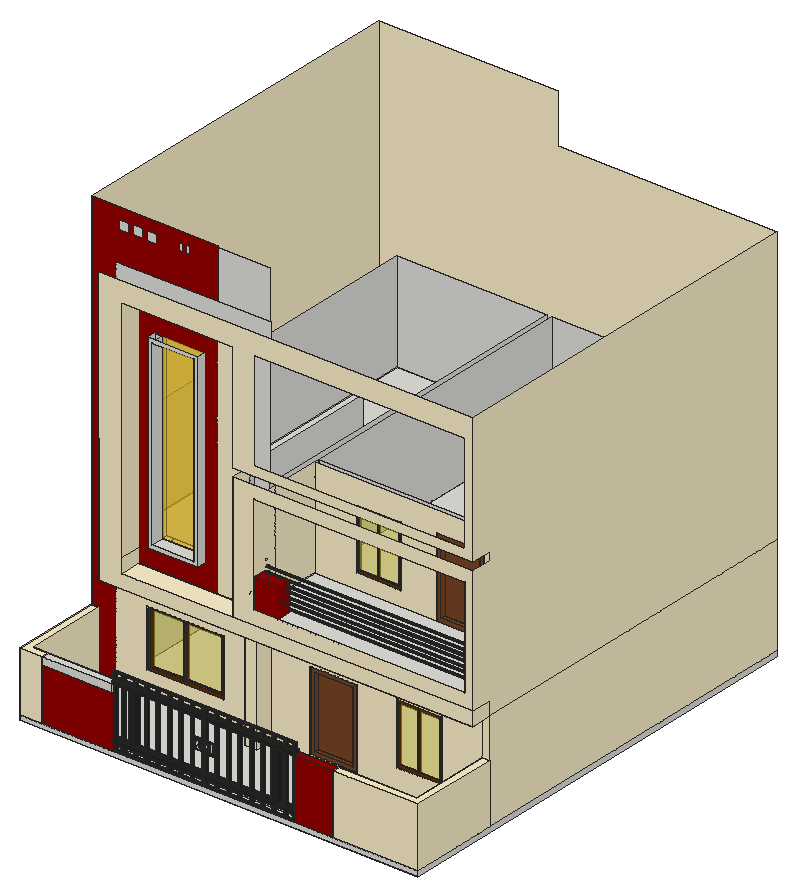
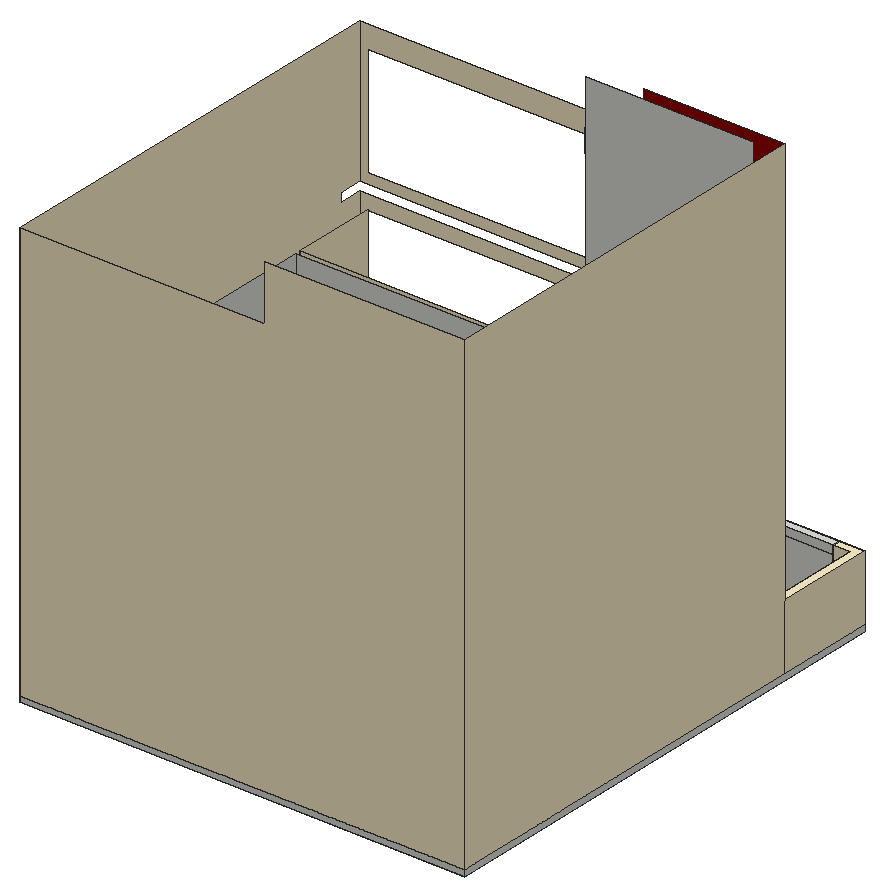
# SketchUp Ruby script. Lengths in inches.
U = 1.inch
M = Sketchup.active_model
def pt(a) = Geom::Point3d.new(a.map { |v| v * U })
def face(e, loops, mat)
  f = e.add_face(loops[0].map { |a| pt(a) })
  loops[1..].each { |l| e.add_face(l.map { |a| pt(a) }).erase! }
  f.material = f.back_material = mat if mat
  f
end
# faces: each face lists its corners as indices into pts; further lists are holes
def faces(e, pts, list, mat = nil) = list.each { |f| face(e, (f[0].is_a?(Array) ? f : [f]).map { |l| l.map { |i| pts[i] } }, mat) }
# xy, xz, yz: faces in a plane at the given z, y or x. An outline is a flat list of corners, or four numbers for a rectangle; further outlines are holes
def ring(l) = l.size == 4 ? [[l[0], l[1]], [l[2], l[1]], [l[2], l[3]], [l[0], l[3]]] : l.each_slice(2).to_a
def flat(e, list, mat, &to3) = list.each { |f| face(e, (f[0].is_a?(Array) ? f : [f]).map { |l| ring(l).map { |u, v| to3.(u, v) } }, mat) }
def xy(e, z, list, mat = nil) = flat(e, list, mat) { |x, y| [x, y, z] }
def xz(e, y, list, mat = nil) = flat(e, list, mat) { |x, z| [x, y, z] }
def yz(e, x, list, mat = nil) = flat(e, list, mat) { |y, z| [x, y, z] }
def lines(e, pts, list) = list.each { |a, b| e.add_line(pt(pts[a]), pt(pts[b])) }
# prism: a flat outline (further loops are holes) pulled along v
def prism(e, loops, v, mat = nil)
  f = face(e, loops, mat); d = Geom::Vector3d.new(v.map { |x| x * U })
  f.pushpull(f.normal.samedirection?(d) ? d.length : -d.length)
end
def box(e, o, s, mat = nil) = prism(e, [[o, [o[0] + s[0], o[1], o[2]], [o[0] + s[0], o[1] + s[1], o[2]], [o[0], o[1] + s[1], o[2]]]], [0, 0, s[2]], mat)
def at(x, y, z, deg = 0) = Geom::Transformation.translation(pt([x, y, z])) * Geom::Transformation.rotation(ORIGIN, Z_AXIS, deg.degrees)
def axes(o, x, y, z) = Geom::Transformation.new([*x, 0, *y, 0, *z, 0, *pt(o).to_a, 1])
def part(name) = M.definitions.add(name)
# library, detail: a bought-in or finely detailed component or shape, given as its bounding box
def library(name, o, s) = part(name).tap { |d| box(d.entities, o, s) }
def detail(e, o, s) = box(e.add_group.entities, o, s)
def put(e, d, t, mat = nil) = e.add_instance(d, t).tap { |i| i.material = mat if mat }
def group(e, t, mat = nil) = e.add_group.tap { |g| g.transformation = t; g.material = mat if mat }.entities
root = M.entities
M.materials.add("[Color A07]").color = [153, 0, 0]
M.materials.add("[Color C08]").color = [102, 51, 0]
M.materials.add("[Color D01]").color = [255, 242, 204]
M.materials.add("[Color M00]").color = [255, 255, 255]
M.materials.add("[Color M09]").color = [0, 0, 0]
M.materials.add("[Metal Corrugated Shiny]").color = [38, 38, 38]
M.materials.add("[Metal Silver]").color = [234, 233, 238]
M.materials.add("[Translucent Glass Blue]").color = [253, 204, 30]
M.materials["[Translucent Glass Blue]"].alpha = 0.5
M.materials.add("[Translucent Glass Gray]").color = [238, 223, 60]
M.materials["[Translucent Glass Gray]"].alpha = 0.5
M.materials.add("[Wood Veneer 01]").color = [120, 70, 37]
c1 = part("Component\#24")
prism(c1.entities,[[[0,1.89,1.72],[0,1.6875,1.91],[0,1.44,2.04],[0,1.18,2.11],[0,0.9,2.11],[0,0.63,2.03],[0,0.39,1.89],[0,0.2,1.6875],[0,0.07,1.44],[0,0,1.18],[0,0,0.9],[0,0.08,0.63],[0,0.22,0.39],[0,0.42,0.2],[0,0.67,0.07],[0,0.9375,0],[0,1.21,0],[0,1.48,0.08],[0,1.72,0.22],[0,1.91,0.42],[0,2.04,0.67],[0,2.11,0.9375],[0,2.11,1.21],[0,2.03,1.48]]],[-0.625,0,0])
c2 = part("Gate cross rail")
box(c2.entities,[0,0,0],[3,48,2])
c3 = part("Gate edge rail")
box(c3.entities,[0,0.5625,0],[48,0.625,0.625])
c4 = part("Gate picket")
box(c4.entities,[0,0,0],[63,1.1875,0.625])
c5 = part("Gate rail")
box(c5.entities,[0,0,0],[3,45,2])
c6 = part("Component\#23")
xy(c6.entities,0,[[0,0,11.01,4.67]])
c7 = part("Gate grille")
put(c7.entities,c2,at(54.625,0,0),"[Metal Corrugated Shiny]")
put(c7.entities,c3,axes([0.625,0,1.96],[0,1,0],[0,0,-1],[-1,0,0]),"[Metal Corrugated Shiny]")
put(c7.entities,c4,at(0.625,46.8125,0.78),"[Metal Corrugated Shiny]")
put(c7.entities,c2,at(6.625,0,0),"[Metal Corrugated Shiny]")
put(c7.entities,c4,at(0.625,10.8125,0.78),"[Metal Corrugated Shiny]")
put(c7.entities,c4,at(0.625,4.8125,0.78),"[Metal Corrugated Shiny]")
put(c7.entities,c3,axes([64.25,0,1.96],[0,1,0],[0,0,-1],[-1,0,0]),"[Metal Corrugated Shiny]")
put(c7.entities,c4,at(0.625,34.8125,0.78),"[Metal Corrugated Shiny]")
put(c7.entities,c4,at(0.625,28.8125,0.78),"[Metal Corrugated Shiny]")
put(c7.entities,c4,at(0.625,40.8125,0.78),"[Metal Corrugated Shiny]")
put(c7.entities,c5,at(9.625,12,0,-90),"[Metal Corrugated Shiny]")
put(c7.entities,c4,at(0.625,22.8125,0.78),"[Metal Corrugated Shiny]")
put(c7.entities,c4,at(0.625,0,0.78),"[Metal Corrugated Shiny]")
put(c7.entities,c4,at(0.625,16.8125,0.78),"[Metal Corrugated Shiny]")
put(c7.entities,c6,axes([26.47,42,1.4],[1,0,0],[0,1.14286,0],[0,0,1]),"[Metal Corrugated Shiny]")
c8 = part("Component\#25")
box(c8.entities,[-0.625,0,0],[0.625,0.9375,5.875])
c9 = part("Forecourt gate leaf")
put(c9.entities,c1,at(0.625,39.09,32.62),"[Metal Silver]")
put(c9.entities,c7,axes([2.03,0,0],[0,0,1],[0,0.875,0],[-1,0,0]))
put(c9.entities,c8,at(0.625,38.15,29.71),"[Metal Silver]")
c10 = part("Group\#2")
xy(c10.entities,0,[[0,0,48,5.9375]],"[Wood Veneer 01]")
xy(c10.entities,4.11,[[4.11,0,43.89,5.9375]],"[Wood Veneer 01]")
xy(c10.entities,79.89,[[4.11,0,43.89,5.9375]],"[Wood Veneer 01]")
xy(c10.entities,84,[[0,0,48,5.9375]],"[Wood Veneer 01]")
xz(c10.entities,0,[[[0,0,48,84],[4.11,4.11,43.89,79.89]]],"[Wood Veneer 01]")
xz(c10.entities,5.9375,[[[0,0,48,84],[4.11,4.11,43.89,79.89]],[4.11,4.11,43.89,79.89]],"[Wood Veneer 01]")
yz(c10.entities,0,[[0,0,5.9375,84]],"[Wood Veneer 01]")
yz(c10.entities,4.11,[[0,4.11,5.9375,79.89]],"[Wood Veneer 01]")
yz(c10.entities,43.89,[[0,4.11,5.9375,79.89]],"[Wood Veneer 01]")
yz(c10.entities,48,[[0,0,5.9375,84]],"[Wood Veneer 01]")
c11 = part("Group\#1")
xy(c11.entities,0,[[0,0,119.6875,5.25]],"[Color C08]")
xy(c11.entities,5.1875,[[5.1875,0,56.1875,5.25],[56.1875,0,59.84,5.25],[59.84,0,114.5,5.25]],"[Color C08]")
xy(c11.entities,114.5,[[5.1875,0,56.1875,5.25],[56.1875,0,59.84,5.25],[59.84,0,114.5,5.25]],"[Color C08]")
xy(c11.entities,119.6875,[[0,0,119.6875,5.25]],"[Color C08]")
xz(c11.entities,0,[[[0,0,119.6875,119.6875],[5.1875,5.1875,114.5,114.5]],[56.1875,5.1875,59.84,114.5]],"[Color C08]")
xz(c11.entities,0,[[5.1875,5.1875,56.1875,114.5],[59.84,5.1875,114.5,114.5]],"[Translucent Glass Gray]")
xz(c11.entities,5.25,[[[0,0,119.6875,119.6875],[5.1875,5.1875,114.5,114.5]],[56.1875,5.1875,59.84,114.5]],"[Color C08]")
yz(c11.entities,0,[[0,0,5.25,119.6875]],"[Color C08]")
yz(c11.entities,5.1875,[[0,5.1875,5.25,114.5]],"[Color C08]")
yz(c11.entities,56.1875,[[0,5.1875,5.25,114.5]],"[Color C08]")
yz(c11.entities,59.84,[[0,5.1875,5.25,114.5]],"[Color C08]")
yz(c11.entities,114.5,[[0,5.1875,5.25,114.5]],"[Color C08]")
yz(c11.entities,119.6875,[[0,0,5.25,119.6875]],"[Color C08]")
xy(root,0,[[0,0.625,480,540.625]])
xy(root,6,[[0,0.625,0,108.25,9,108.25,9,9.625,26.71,9.625,26.71,0.625],[26.71,0.625,110.46,9.625],[110.46,0.625,329.85,9.625],[329.85,0.625,377.41,9.625],[377.41,0.625,377.41,9.625,471,9.625,471,108.25,480,108.25,480,0.625],
  [9,9.625,471,9.625,471,108.25,215.91,108.25,215.91,86.8125,201.94,86.8125,201.94,108.25,9,108.25],[[0,108.25,480,540.625],[216.3125,114.25,471,531.625],[29.875,114.25,210.3125,531.625]],[29.875,114.25,210.3125,531.625],[216.3125,114.25,471,531.625]])
xy(root,8.27,[[262.79,108.25,319.98,114.25]])
xy(root,30.65,[[66.9,108.25,160.09,114.25]])
xy(root,31.26,[[368.53,108.25,422.35,114.25]])
xy(root,68.9375,[[26.71,0.625,110.46,9.625]])
xy(root,78,[[26.71,0.625,110.46,9.625]])
xy(root,78,[[329.85,0.625,377.41,9.625]],"[Color A07]")
xy(root,78,[[0,0.625,26.71,0.625,26.71,9.625,9,9.625,9,108.25,0,108.25],[377.41,0.625,480,0.625,480,108.25,471,108.25,471,9.625,377.41,9.625]],"[Color D01]")
xy(root,100.15,[[66.9,108.25,160.09,114.25]])
xy(root,103.83,[[262.79,108.25,319.98,114.25]])
xy(root,105.07,[[368.53,108.25,422.35,114.25]])
xy(root,126,[[471,82.5625,480,108.25],[201.94,86.8125,215.91,108.25]])
xy(root,126,[[29.875,82.5625,471,82.5625,471,108.25,215.91,108.25,215.91,86.8125,201.94,86.8125,201.94,108.25,29.875,108.25]],"[Color M00]")
xy(root,142.4375,[[191.1875,82.5625,471,108.25],[471,82.5625,480,108.25],[191.1875,108.25,471,278.125]])
xy(root,142.4375,[[56.54,82.5625,191.1875,108.25]],"[Color D01]")
xy(root,152.875,[[29.875,114.25,210.3125,531.625],[216.3125,114.25,471,531.625]])
xy(root,158.875,[[245.1875,82.5625,471,82.5625,471,114.25,216.3125,114.25,216.3125,98.41,245.1875,98.41],[29.875,114.25,210.3125,531.625],[216.3125,114.25,471,114.25,471,173.875,420.42,173.875,420.42,179.875,363.24,179.875,363.24,173.875,216.3125,173.875],[216.3125,173.875,363.24,179.875],[420.42,173.875,471,179.875],
  [216.3125,179.875,471,531.625]])
xy(root,158.875,[[216.3125,82.5625,245.1875,98.41]],"[Color A07]")
xy(root,170.55,[[76.39,97.9375,136.32,108.25]])
xy(root,174.89,[[80.73,97.9375,131.98,114.25]])
xy(root,174.89,[[80.73,114.25,90.73,120.5625],[90.73,114.25,131.98,120.5625]],"[Translucent Glass Blue]")
xy(root,176.66,[[266.86,173.875,320.67,179.875]])
xy(root,194.875,[[216.3125,82.5625,245.1875,98.41]],"[Color A07]")
xz(root,0.625,[[0,0,480,6],[26.71,68.9375,110.46,78]])
xz(root,0.625,[[26.71,6,110.46,68.9375],[329.85,6,377.41,78]],"[Color A07]")
xz(root,0.625,[[0,6,26.71,78],[377.41,6,480,78]],"[Color D01]")
xz(root,9.625,[[26.71,6,110.46,68.9375],[329.85,6,377.41,78],[26.71,68.9375,110.46,78]])
xz(root,9.625,[[9,6,26.71,78],[377.41,6,471,78]],"[Color D01]")
xz(root,82.5625,[[216.3125,158.875,245.1875,194.875]],"[Color A07]")
xz(root,82.5625,[[[29.875,126,480,126,480,142.4375,56.54,142.4375,56.54,434.875,191.1875,434.875,191.1875,303.625,480,303.625,480,458.875,29.875,458.875],[216.3125,314.875,471,434.875]],[[191.1875,142.4375,480,293.6875],[216.3125,158.875,471,278.875]]],"[Color D01]")
xz(root,86.8125,[[201.94,6,215.91,126]],"[Color D01]")
xz(root,97.9375,[[[76.39,170.55,136.32,397.86],[80.73,174.89,131.98,393.52]]])
xz(root,98.41,[[216.3125,158.875,245.1875,194.875]],"[Color A07]")
xz(root,108.25,[[0,6,9,78],[201.94,6,215.91,126],[471,6,480,78],[29.875,126,29.875,458.875,216.3125,458.875,216.3125,434.875,56.54,434.875,56.54,142.4375,480,142.4375,480,126]])
xz(root,108.25,[[[9,6,29.875,6,29.875,458.875,152.27,458.875,152.27,518.875,0,518.875,0,78,9,78],[66.875,493.93,79,506.06],[33.0625,493.93,45.1875,506.06],[49.25,493.93,61.375,506.06],[105.77,497.1,110.39,506.41],[113.89,497.1,118.52,506.41]],[[56.54,142.4375,151.34,434.875],[76.39,170.55,136.32,397.86]]],"[Color A07]")
xz(root,108.25,[[[29.875,6,201.94,126],[66.9,30.65,160.09,100.15]],[[215.91,6,471,126],[262.79,8.27,319.98,103.83],[368.53,31.26,422.35,105.07]],[471,78,480,126],[151.34,142.4375,191.1875,434.875]],"[Color D01]")
xz(root,114.25,[[[29.875,6,210.3125,126],[66.9,30.65,160.09,100.15]],[[216.3125,6,471,126],[262.79,8.27,319.98,103.83],[368.53,31.26,422.35,105.07]],[29.875,126,210.3125,152.875],[216.3125,126,471,152.875],[29.875,152.875,210.3125,158.875],
  [216.3125,152.875,471,158.875],[[29.875,158.875,210.3125,512.875],[80.73,174.89,131.98,393.52]]])
xz(root,114.25,[[80.73,174.89,131.98,393.52]],"[Translucent Glass Blue]")
xz(root,120.5625,[[80.73,174.89,131.98,393.52]],"[Translucent Glass Blue]")
xz(root,173.875,[[[216.3125,158.875,363.24,158.875,363.24,254.4375,420.42,254.4375,420.42,158.875,471,158.875,471,278.875,216.3125,278.875],[266.86,176.66,320.67,250.47]]],"[Color D01]")
xz(root,179.875,[[[216.3125,158.875,216.3125,278.875,471,278.875,471,158.875,420.42,158.875,420.42,254.4375,363.24,254.4375,363.24,158.875],[266.86,176.66,320.67,250.47]]])
xz(root,531.625,[[29.875,6,210.3125,126],[216.3125,6,471,126],[29.875,126,210.3125,152.875],[216.3125,126,471,152.875],[29.875,152.875,44,158.875],
  [44,152.875,210.3125,158.875],[216.3125,152.875,243.11,158.875],[243.11,152.875,283.49,158.875],[283.49,152.875,471,158.875],[29.875,158.875,210.3125,278.875],
  [216.3125,158.875,471,278.875]])
xz(root,540.625,[[0,0,480,6]])
xz(root,540.625,[[0,6,0,518.875,216.3125,518.875,216.3125,458.875,480,458.875,480,6]],"[Color D01]")
yz(root,0,[[0.625,0,540.625,6]])
yz(root,0,[[0.625,6,108.25,78],[108.25,6,540.625,518.875]],"[Color D01]")
yz(root,9,[[9.625,6,108.25,78]],"[Color D01]")
yz(root,26.71,[[0.625,6,9.625,68.9375],[0.625,68.9375,9.625,78]])
yz(root,29.875,[[114.25,6,531.625,126],[108.25,126,114.25,158.875],[114.25,126,531.625,152.875],[114.25,152.875,531.625,158.875],[108.25,158.875,114.25,278.875],
  [114.25,158.875,531.625,278.875]])
yz(root,29.875,[[82.5625,126,108.25,158.875],[82.5625,158.875,108.25,278.875]],"[Color D01]")
yz(root,56.54,[[82.5625,142.4375,108.25,158.875],[82.5625,158.875,108.25,434.875]],"[Color D01]")
yz(root,66.9,[[108.25,30.65,114.25,100.15]])
yz(root,76.39,[[97.9375,170.55,108.25,397.86]])
yz(root,80.73,[[97.9375,174.89,114.25,393.52]])
yz(root,80.73,[[114.25,174.89,120.5625,393.52]],"[Translucent Glass Blue]")
yz(root,110.46,[[0.625,68.9375,9.625,78]])
yz(root,110.46,[[0.625,6,9.625,68.9375]],"[Color A07]")
yz(root,131.98,[[97.9375,174.89,114.25,393.52]])
yz(root,131.98,[[114.25,174.89,120.5625,393.52]],"[Translucent Glass Blue]")
yz(root,136.32,[[97.9375,170.55,108.25,397.86]])
yz(root,160.09,[[108.25,30.65,114.25,100.15]])
yz(root,191.1875,[[108.25,142.4375,278.125,296.875]])
yz(root,191.1875,[[82.5625,142.4375,108.25,293.6875]],"[Color D01]")
yz(root,194.625,[[100.96,160.84,100.68,160.875,100.43,160.98,100.21,161.15,100.04,161.37,99.93,161.63,99.9,161.9,99.93,162.18,100.04,162.43,100.21,162.65,100.43,162.82,100.68,162.93,100.96,162.97,101.23,162.93,101.49,162.82,101.71,162.65,101.88,162.43,101.99,162.18,102.02,161.9,101.99,161.63,101.88,161.37,101.71,161.15,101.49,160.98,101.23,160.875]],"[Color M09]")
yz(root,201.94,[[86.8125,6,108.25,126]],"[Color D01]")
yz(root,210.3125,[[114.25,6,531.625,126],[114.25,126,531.625,152.875],[114.25,152.875,531.625,158.875],[114.25,158.875,531.625,278.875]])
yz(root,215.91,[[86.8125,6,108.25,126]],"[Color D01]")
yz(root,216.3125,[[114.25,6,531.625,126],[114.25,126,531.625,152.875],[114.25,152.875,531.625,158.875],[173.875,158.875,179.875,278.875],[179.875,158.875,531.625,278.875]])
yz(root,216.3125,[[82.5625,158.875,98.41,194.875]],"[Color A07]")
yz(root,216.3125,[[[98.41,158.875,114.25,158.875,114.25,278.875,82.5625,278.875,82.5625,194.875,98.41,194.875],[98.41,203.98,103.375,206.875],[100.96,197.22,100.68,197.25,100.43,197.36,100.21,197.53,100.04,197.75,99.93,198,99.9,198.28,99.93,198.55,100.04,198.81,100.21,199.03,100.43,199.2,100.68,199.3,100.96,199.34,101.23,199.3,101.49,199.2,101.71,199.03,101.88,198.81,101.99,198.55,102.02,198.28,101.99,198,101.88,197.75,101.71,197.53,101.49,197.36,101.23,197.25],[100.96,191.15,100.68,191.1875,100.43,191.3,100.21,191.46,100.04,191.68,99.93,191.94,99.9,192.22,99.93,192.49,100.04,192.75,100.21,192.97,100.43,193.14,100.68,193.24,100.96,193.28,101.23,193.24,101.49,193.14,101.71,192.97,101.88,192.75,101.99,192.49,102.02,192.22,101.99,191.94,101.88,191.68,101.71,191.46,101.49,191.3,101.23,191.1875],[100.96,185.09,100.68,185.125,100.43,185.23,100.21,185.4,100.04,185.62,99.93,185.88,99.9,186.15,99.93,186.43,100.04,186.68,100.21,186.9,100.43,187.07,100.68,187.18,100.96,187.22,101.23,187.18,101.49,187.07,101.71,186.9,101.88,186.68,101.99,186.43,102.02,186.15,101.99,185.88,101.88,185.62,101.71,185.4,101.49,185.23,101.23,185.125],[100.96,172.97,100.68,173,100.43,173.11,100.21,173.28,100.04,173.5,99.93,173.75,99.9,174.03,99.93,174.3,100.04,174.56,100.21,174.78,100.43,174.95,100.68,175.05,100.96,175.09,101.23,175.05,101.49,174.95,101.71,174.78,101.88,174.56,101.99,174.3,102.02,174.03,101.99,173.75,101.88,173.5,101.71,173.28,101.49,173.11,101.23,173]],[114.25,158.875,173.875,278.875]],"[Color D01]")
yz(root,234,[[100.96,166.9,100.68,166.9375,100.43,167.05,100.21,167.21,100.04,167.43,99.93,167.69,99.9,167.97,99.93,168.24,100.04,168.5,100.21,168.72,100.43,168.89,100.68,168.99,100.96,169.03,101.23,168.99,101.49,168.89,101.71,168.72,101.88,168.5,101.99,168.24,102.02,167.97,101.99,167.69,101.88,167.43,101.71,167.21,101.49,167.05,101.23,166.9375]],"[Color M09]")
yz(root,241.0625,[[100.96,179.03,100.68,179.0625,100.43,179.17,100.21,179.34,100.04,179.56,99.93,179.82,99.9,180.09,99.93,180.37,100.04,180.62,100.21,180.84,100.43,181.01,100.68,181.12,100.96,181.15,101.23,181.12,101.49,181.01,101.71,180.84,101.88,180.62,101.99,180.37,102.02,180.09,101.99,179.82,101.88,179.56,101.71,179.34,101.49,179.17,101.23,179.0625]],"[Color M09]")
yz(root,245.1875,[[82.5625,158.875,98.41,194.875]],"[Color A07]")
yz(root,262.79,[[108.25,8.27,114.25,103.83]])
yz(root,266.86,[[173.875,176.66,179.875,250.47]])
yz(root,319.98,[[108.25,8.27,114.25,103.83]])
yz(root,320.67,[[173.875,176.66,179.875,250.47]])
yz(root,329.85,[[0.625,6,9.625,78]],"[Color A07]")
yz(root,363.24,[[173.875,158.875,179.875,254.4375]])
yz(root,368.53,[[108.25,31.26,114.25,105.07]])
yz(root,377.41,[[0.625,6,9.625,78]])
yz(root,420.42,[[173.875,158.875,179.875,254.4375]])
yz(root,422.35,[[108.25,31.26,114.25,105.07]])
yz(root,471,[[114.25,6,531.625,126],[114.25,126,114.25,142.4375,278.125,142.4375,278.125,152.875,531.625,152.875,531.625,126],[114.25,142.4375,278.125,152.875],[114.25,152.875,278.125,158.875],[100.96,154.78,101.23,154.8125,101.49,154.92,101.71,155.09,101.88,155.31,101.99,155.57,102.02,155.84,101.99,156.12,101.88,156.37,101.71,156.59,101.49,156.76,101.23,156.87,100.96,156.9,100.68,156.87,100.43,156.76,100.21,156.59,100.04,156.37,99.93,156.12,99.9,155.84,99.93,155.57,100.04,155.31,100.21,155.09,100.43,154.92,100.68,154.8125],
  [[98.41,158.875,103.375,203.98],[100.96,197.22,101.23,197.25,101.49,197.36,101.71,197.53,101.88,197.75,101.99,198,102.02,198.28,101.99,198.55,101.88,198.81,101.71,199.03,101.49,199.2,101.23,199.3,100.96,199.34,100.68,199.3,100.43,199.2,100.21,199.03,100.04,198.81,99.93,198.55,99.9,198.28,99.93,198,100.04,197.75,100.21,197.53,100.43,197.36,100.68,197.25],[100.96,191.15,101.23,191.1875,101.49,191.3,101.71,191.46,101.88,191.68,101.99,191.94,102.02,192.22,101.99,192.49,101.88,192.75,101.71,192.97,101.49,193.14,101.23,193.24,100.96,193.28,100.68,193.24,100.43,193.14,100.21,192.97,100.04,192.75,99.93,192.49,99.9,192.22,99.93,191.94,100.04,191.68,100.21,191.46,100.43,191.3,100.68,191.1875],[100.96,185.09,101.23,185.125,101.49,185.23,101.71,185.4,101.88,185.62,101.99,185.88,102.02,186.15,101.99,186.43,101.88,186.68,101.71,186.9,101.49,187.07,101.23,187.18,100.96,187.22,100.68,187.18,100.43,187.07,100.21,186.9,100.04,186.68,99.93,186.43,99.9,186.15,99.93,185.88,100.04,185.62,100.21,185.4,100.43,185.23,100.68,185.125],[100.96,179.03,101.23,179.0625,101.49,179.17,101.71,179.34,101.88,179.56,101.99,179.82,102.02,180.09,101.99,180.37,101.88,180.62,101.71,180.84,101.49,181.01,101.23,181.12,100.96,181.15,100.68,181.12,100.43,181.01,100.21,180.84,100.04,180.62,99.93,180.37,99.9,180.09,99.93,179.82,100.04,179.56,100.21,179.34,100.43,179.17,100.68,179.0625],[100.96,172.97,101.23,173,101.49,173.11,101.71,173.28,101.88,173.5,101.99,173.75,102.02,174.03,101.99,174.3,101.88,174.56,101.71,174.78,101.49,174.95,101.23,175.05,100.96,175.09,100.68,175.05,100.43,174.95,100.21,174.78,100.04,174.56,99.93,174.3,99.9,174.03,99.93,173.75,100.04,173.5,100.21,173.28,100.43,173.11,100.68,173],[100.96,166.9,101.23,166.9375,101.49,167.05,101.71,167.21,101.88,167.43,101.99,167.69,102.02,167.97,101.99,168.24,101.88,168.5,101.71,168.72,101.49,168.89,101.23,168.99,100.96,169.03,100.68,168.99,100.43,168.89,100.21,168.72,100.04,168.5,99.93,168.24,99.9,167.97,99.93,167.69,100.04,167.43,100.21,167.21,100.43,167.05,100.68,166.9375],[100.96,160.84,101.23,160.875,101.49,160.98,101.71,161.15,101.88,161.37,101.99,161.63,102.02,161.9,101.99,162.18,101.88,162.43,101.71,162.65,101.49,162.82,101.23,162.93,100.96,162.97,100.68,162.93,100.43,162.82,100.21,162.65,100.04,162.43,99.93,162.18,99.9,161.9,99.93,161.63,100.04,161.37,100.21,161.15,100.43,160.98,100.68,160.875]],[179.875,158.875,531.625,278.875]])
yz(root,471,[[9.625,6,108.25,78],[82.5625,158.875,82.5625,278.875,173.875,278.875,173.875,158.875,103.375,158.875,103.375,206.875,98.41,206.875,98.41,158.875]],"[Color D01]")
yz(root,471,[[100.96,191.15,101.23,191.1875,101.49,191.3,101.71,191.46,101.88,191.68,101.99,191.94,102.02,192.22,101.99,192.49,101.88,192.75,101.71,192.97,101.49,193.14,101.23,193.24,100.96,193.28,100.68,193.24,100.43,193.14,100.21,192.97,100.04,192.75,99.93,192.49,99.9,192.22,99.93,191.94,100.04,191.68,100.21,191.46,100.43,191.3,100.68,191.1875],[100.96,197.22,101.23,197.25,101.49,197.36,101.71,197.53,101.88,197.75,101.99,198,102.02,198.28,101.99,198.55,101.88,198.81,101.71,199.03,101.49,199.2,101.23,199.3,100.96,199.34,100.68,199.3,100.43,199.2,100.21,199.03,100.04,198.81,99.93,198.55,99.9,198.28,99.93,198,100.04,197.75,100.21,197.53,100.43,197.36,100.68,197.25]],"[Color M09]")
yz(root,480,[[0.625,0,540.625,6]])
yz(root,480,[[0.625,6,108.25,78],[108.25,6,540.625,126],[108.25,126,540.625,126,540.625,458.875,82.5625,458.875,82.5625,303.625,108.25,303.625,108.25,293.6875,82.5625,293.6875,82.5625,142.4375,108.25,142.4375],[82.5625,126,108.25,142.4375]],"[Color D01]")
p = [[471,100.96,160.84],[471,100.68,160.875],[194.625,100.68,160.875],[194.625,100.96,160.84],[471,101.23,160.875],[194.625,101.23,160.875],
  [471,100.43,160.98],[194.625,100.43,160.98],[471,101.49,160.98],[194.625,101.49,160.98],[471,100.21,161.15],[194.625,100.21,161.15],
  [471,101.71,161.15],[194.625,101.71,161.15],[471,100.04,161.37],[194.625,100.04,161.37],[471,101.88,161.37],[194.625,101.88,161.37],
  [471,99.93,161.63],[194.625,99.93,161.63],[471,101.99,161.63],[194.625,101.99,161.63],[471,99.9,161.9],[194.625,99.9,161.9],
  [471,102.02,161.9],[194.625,102.02,161.9],[471,99.93,162.18],[194.625,99.93,162.18],[471,101.99,162.18],[194.625,101.99,162.18],
  [471,100.04,162.43],[194.625,100.04,162.43],[471,101.88,162.43],[194.625,101.88,162.43],[471,100.21,162.65],[194.625,100.21,162.65],
  [471,101.71,162.65],[194.625,101.71,162.65],[471,100.43,162.82],[194.625,100.43,162.82],[471,101.49,162.82],[194.625,101.49,162.82],
  [471,100.68,162.93],[194.625,100.68,162.93],[471,101.23,162.93],[194.625,101.23,162.93],[471,100.96,162.97],[194.625,100.96,162.97],
  [471,100.68,166.9375],[471,100.43,167.05],[234,100.43,167.05],[234,100.68,166.9375],[471,100.96,166.9],[234,100.96,166.9],
  [471,101.23,166.9375],[234,101.23,166.9375],[471,101.49,167.05],[234,101.49,167.05],[471,100.21,167.21],[234,100.21,167.21],
  [471,101.71,167.21],[234,101.71,167.21],[471,100.04,167.43],[234,100.04,167.43],[471,101.88,167.43],[234,101.88,167.43],
  [471,99.93,167.69],[234,99.93,167.69],[471,101.99,167.69],[234,101.99,167.69],[471,99.9,167.97],[234,99.9,167.97],
  [471,102.02,167.97],[234,102.02,167.97],[471,99.93,168.24],[234,99.93,168.24],[471,101.99,168.24],[234,101.99,168.24],
  [471,100.04,168.5],[234,100.04,168.5],[471,101.88,168.5],[234,101.88,168.5],[471,100.21,168.72],[234,100.21,168.72],
  [471,101.71,168.72],[234,101.71,168.72],[471,100.43,168.89],[234,100.43,168.89],[471,101.49,168.89],[234,101.49,168.89],
  [471,100.68,168.99],[234,100.68,168.99],[471,101.23,168.99],[234,101.23,168.99],[471,100.96,169.03],[234,100.96,169.03],
  [471,100.68,173],[471,100.43,173.11],[216.3125,100.43,173.11],[216.3125,100.68,173],[471,100.96,172.97],[216.3125,100.96,172.97],
  [471,101.23,173],[216.3125,101.23,173],[471,101.49,173.11],[216.3125,101.49,173.11],[471,100.21,173.28],[216.3125,100.21,173.28],
  [471,101.71,173.28],[216.3125,101.71,173.28],[471,100.04,173.5],[216.3125,100.04,173.5],[471,101.88,173.5],[216.3125,101.88,173.5],
  [471,99.93,173.75],[216.3125,99.93,173.75],[471,101.99,173.75],[216.3125,101.99,173.75],[471,99.9,174.03],[216.3125,99.9,174.03],
  [471,102.02,174.03],[216.3125,102.02,174.03],[471,99.93,174.3],[216.3125,99.93,174.3],[471,101.99,174.3],[216.3125,101.99,174.3],
  [471,100.04,174.56],[216.3125,100.04,174.56],[471,101.88,174.56],[216.3125,101.88,174.56],[471,100.21,174.78],[216.3125,100.21,174.78],
  [471,101.71,174.78],[216.3125,101.71,174.78],[471,100.43,174.95],[216.3125,100.43,174.95],[471,101.49,174.95],[216.3125,101.49,174.95],
  [471,100.68,175.05],[216.3125,100.68,175.05],[471,101.23,175.05],[216.3125,101.23,175.05],[471,100.96,175.09],[216.3125,100.96,175.09],
  [471,100.96,179.03],[471,100.68,179.0625],[241.0625,100.68,179.0625],[241.0625,100.96,179.03],[471,101.23,179.0625],[241.0625,101.23,179.0625],
  [471,100.43,179.17],[241.0625,100.43,179.17],[471,101.49,179.17],[241.0625,101.49,179.17],[471,100.21,179.34],[241.0625,100.21,179.34],
  [471,101.71,179.34],[241.0625,101.71,179.34],[471,100.04,179.56],[241.0625,100.04,179.56],[471,101.88,179.56],[241.0625,101.88,179.56],
  [471,99.93,179.82],[241.0625,99.93,179.82],[471,101.99,179.82],[241.0625,101.99,179.82],[471,99.9,180.09],[241.0625,99.9,180.09],
  [471,102.02,180.09],[241.0625,102.02,180.09],[471,99.93,180.37],[241.0625,99.93,180.37],[471,101.99,180.37],[241.0625,101.99,180.37],
  [471,100.04,180.62],[241.0625,100.04,180.62],[471,101.88,180.62],[241.0625,101.88,180.62],[471,100.21,180.84],[241.0625,100.21,180.84],
  [471,101.71,180.84],[241.0625,101.71,180.84],[471,100.43,181.01],[241.0625,100.43,181.01],[471,101.49,181.01],[241.0625,101.49,181.01],
  [471,100.68,181.12],[241.0625,100.68,181.12],[471,101.23,181.12],[241.0625,101.23,181.12],[471,100.96,181.15],[241.0625,100.96,181.15],
  [471,100.68,185.125],[471,100.43,185.23],[216.3125,100.43,185.23],[216.3125,100.68,185.125],[471,100.96,185.09],[216.3125,100.96,185.09],
  [471,101.23,185.125],[216.3125,101.23,185.125],[471,101.49,185.23],[216.3125,101.49,185.23],[471,100.21,185.4],[216.3125,100.21,185.4],
  [471,101.71,185.4],[216.3125,101.71,185.4],[471,100.04,185.62],[216.3125,100.04,185.62],[471,101.88,185.62],[216.3125,101.88,185.62],
  [471,99.93,185.88],[216.3125,99.93,185.88],[471,101.99,185.88],[216.3125,101.99,185.88],[471,99.9,186.15],[216.3125,99.9,186.15],
  [471,102.02,186.15],[216.3125,102.02,186.15],[471,99.93,186.43],[216.3125,99.93,186.43],[471,101.99,186.43],[216.3125,101.99,186.43],
  [471,100.04,186.68],[216.3125,100.04,186.68],[471,101.88,186.68],[216.3125,101.88,186.68],[471,100.21,186.9],[216.3125,100.21,186.9],
  [471,101.71,186.9],[216.3125,101.71,186.9],[471,100.43,187.07],[216.3125,100.43,187.07],[471,101.49,187.07],[216.3125,101.49,187.07],
  [471,100.68,187.18],[216.3125,100.68,187.18],[471,101.23,187.18],[216.3125,101.23,187.18],[471,100.96,187.22],[216.3125,100.96,187.22],
  [471,100.68,191.1875],[471,100.43,191.3],[216.3125,100.43,191.3],[216.3125,100.68,191.1875],[471,100.96,191.15],[216.3125,100.96,191.15],
  [471,101.23,191.1875],[216.3125,101.23,191.1875],[471,101.49,191.3],[216.3125,101.49,191.3],[471,100.21,191.46],[216.3125,100.21,191.46],
  [471,101.71,191.46],[216.3125,101.71,191.46],[471,100.04,191.68],[216.3125,100.04,191.68],[471,101.88,191.68],[216.3125,101.88,191.68],
  [471,99.93,191.94],[216.3125,99.93,191.94],[471,101.99,191.94],[216.3125,101.99,191.94],[471,99.9,192.22],[216.3125,99.9,192.22],
  [471,102.02,192.22],[216.3125,102.02,192.22],[471,99.93,192.49],[216.3125,99.93,192.49],[471,101.99,192.49],[216.3125,101.99,192.49],
  [471,100.04,192.75],[216.3125,100.04,192.75],[471,101.88,192.75],[216.3125,101.88,192.75],[471,100.21,192.97],[216.3125,100.21,192.97],
  [471,101.71,192.97],[216.3125,101.71,192.97],[471,100.43,193.14],[216.3125,100.43,193.14],[471,101.49,193.14],[216.3125,101.49,193.14],
  [471,100.68,193.24],[216.3125,100.68,193.24],[471,101.23,193.24],[216.3125,101.23,193.24],[471,100.96,193.28],[216.3125,100.96,193.28],
  [471,100.96,197.22],[471,100.68,197.25],[216.3125,100.68,197.25],[216.3125,100.96,197.22],[471,101.23,197.25],[216.3125,101.23,197.25],
  [471,100.43,197.36],[216.3125,100.43,197.36],[471,101.49,197.36],[216.3125,101.49,197.36],[471,100.21,197.53],[216.3125,100.21,197.53],
  [471,101.71,197.53],[216.3125,101.71,197.53],[471,100.04,197.75],[216.3125,100.04,197.75],[471,101.88,197.75],[216.3125,101.88,197.75],
  [471,99.93,198],[216.3125,99.93,198],[471,101.99,198],[216.3125,101.99,198],[471,99.9,198.28],[216.3125,99.9,198.28],
  [471,102.02,198.28],[216.3125,102.02,198.28],[471,99.93,198.55],[216.3125,99.93,198.55],[471,101.99,198.55],[216.3125,101.99,198.55],
  [471,100.04,198.81],[216.3125,100.04,198.81],[471,101.88,198.81],[216.3125,101.88,198.81],[471,100.21,199.03],[216.3125,100.21,199.03],
  [471,101.71,199.03],[216.3125,101.71,199.03],[471,100.43,199.2],[216.3125,100.43,199.2],[471,101.49,199.2],[216.3125,101.49,199.2],
  [471,100.68,199.3],[216.3125,100.68,199.3],[471,101.23,199.3],[216.3125,101.23,199.3],[471,100.96,199.34],[216.3125,100.96,199.34]]
faces(root,p,[[0,1,2,3],[4,0,3,5],[1,6,7,2],[8,4,5,9],[6,10,11,7],[12,8,9,13],[10,14,15,11],[16,12,13,17],
  [14,18,19,15],[20,16,17,21],[18,22,23,19],[24,20,21,25],[22,26,27,23],[28,24,25,29],[26,30,31,27],[32,28,29,33],
  [30,34,35,31],[36,32,33,37],[34,38,39,35],[40,36,37,41],[38,42,43,39],[44,40,41,45],[42,46,47,43],[46,44,45,47],
  [48,49,50,51],[52,48,51,53],[54,52,53,55],[56,54,55,57],[49,58,59,50],[60,56,57,61],[58,62,63,59],[64,60,61,65],
  [62,66,67,63],[68,64,65,69],[66,70,71,67],[72,68,69,73],[70,74,75,71],[76,72,73,77],[74,78,79,75],[80,76,77,81],
  [78,82,83,79],[84,80,81,85],[82,86,87,83],[88,84,85,89],[86,90,91,87],[92,88,89,93],[90,94,95,91],[94,92,93,95],
  [96,97,98,99],[100,96,99,101],[102,100,101,103],[104,102,103,105],[97,106,107,98],[108,104,105,109],[106,110,111,107],[112,108,109,113],
  [110,114,115,111],[116,112,113,117],[114,118,119,115],[120,116,117,121],[118,122,123,119],[124,120,121,125],[122,126,127,123],[128,124,125,129],
  [126,130,131,127],[132,128,129,133],[130,134,135,131],[136,132,133,137],[134,138,139,135],[140,136,137,141],[138,142,143,139],[142,140,141,143],
  [144,145,146,147],[148,144,147,149],[145,150,151,146],[152,148,149,153],[150,154,155,151],[156,152,153,157],[154,158,159,155],[160,156,157,161],
  [158,162,163,159],[164,160,161,165],[162,166,167,163],[168,164,165,169],[166,170,171,167],[172,168,169,173],[170,174,175,171],[176,172,173,177],
  [174,178,179,175],[180,176,177,181],[178,182,183,179],[184,180,181,185],[182,186,187,183],[188,184,185,189],[186,190,191,187],[190,188,189,191],
  [192,193,194,195],[196,192,195,197],[198,196,197,199],[200,198,199,201],[193,202,203,194],[204,200,201,205],[202,206,207,203],[208,204,205,209],
  [206,210,211,207],[212,208,209,213],[210,214,215,211],[216,212,213,217],[214,218,219,215],[220,216,217,221],[218,222,223,219],[224,220,221,225],
  [222,226,227,223],[228,224,225,229],[226,230,231,227],[232,228,229,233],[230,234,235,231],[236,232,233,237],[234,238,239,235],[238,236,237,239],
  [240,241,242,243],[244,240,243,245],[246,244,245,247],[248,246,247,249],[241,250,251,242],[252,248,249,253],[250,254,255,251],[256,252,253,257],
  [254,258,259,255],[260,256,257,261],[258,262,263,259],[264,260,261,265],[262,266,267,263],[268,264,265,269],[266,270,271,267],[272,268,269,273],
  [270,274,275,271],[276,272,273,277],[274,278,279,275],[280,276,277,281],[278,282,283,279],[284,280,281,285],[282,286,287,283],[286,284,285,287],
  [288,289,290,291],[292,288,291,293],[289,294,295,290],[296,292,293,297],[294,298,299,295],[300,296,297,301],[298,302,303,299],[304,300,301,305],
  [302,306,307,303],[308,304,305,309],[306,310,311,307],[312,308,309,313],[310,314,315,311],[316,312,313,317],[314,318,319,315],[320,316,317,321],
  [318,322,323,319],[324,320,321,325],[322,326,327,323],[328,324,325,329],[326,330,331,327],[332,328,329,333],[330,334,335,331],[334,332,333,335]],"[Color M09]")
g1 = group(root,at(110.46,0,6))
put(g1,c9,axes([0,0,84.87],[0,4,0],[2.613,0,0],[0,0,-1.3209]))
put(g1,c9,axes([219.39,0,0],[0,4,0],[-2.613,0,0],[0,0,1.3209]))
put(root,c10,axes([263.82,108.25,8.27],[1.17,0,0],[0,1,0],[0,0,1.13765]))
put(root,c11,axes([66.9,113.16,30.65],[0.77859,0,0],[0,-0.69414,0],[0,0,0.58068]))
put(root,c11,axes([368.65,110.29,31.26],[0.44865,0,0],[0,-0.38095,0],[0,0,0.61671]))
put(root,c10,axes([363.24,174.05,158.875],[1.19141,0,0],[0,0.97,0],[0,0,1.13662]))
put(root,c11,axes([266.97,175.875,176.66],[0.44865,0,0],[0,-0.38095,0],[0,0,0.61671]))
